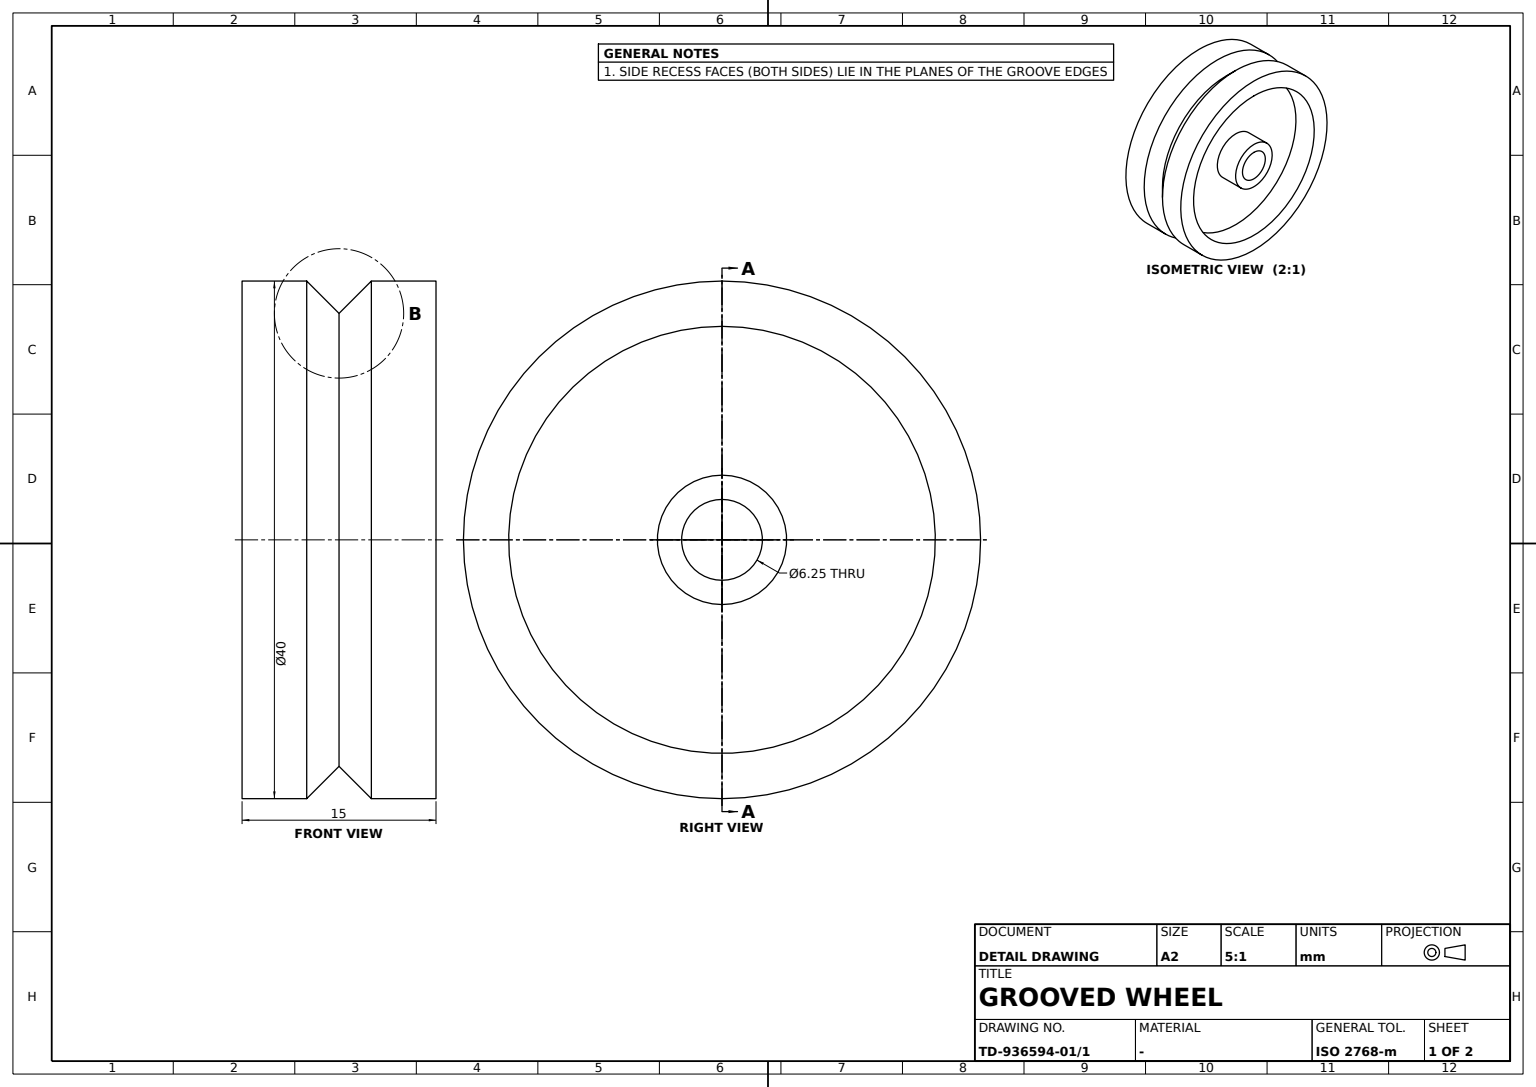
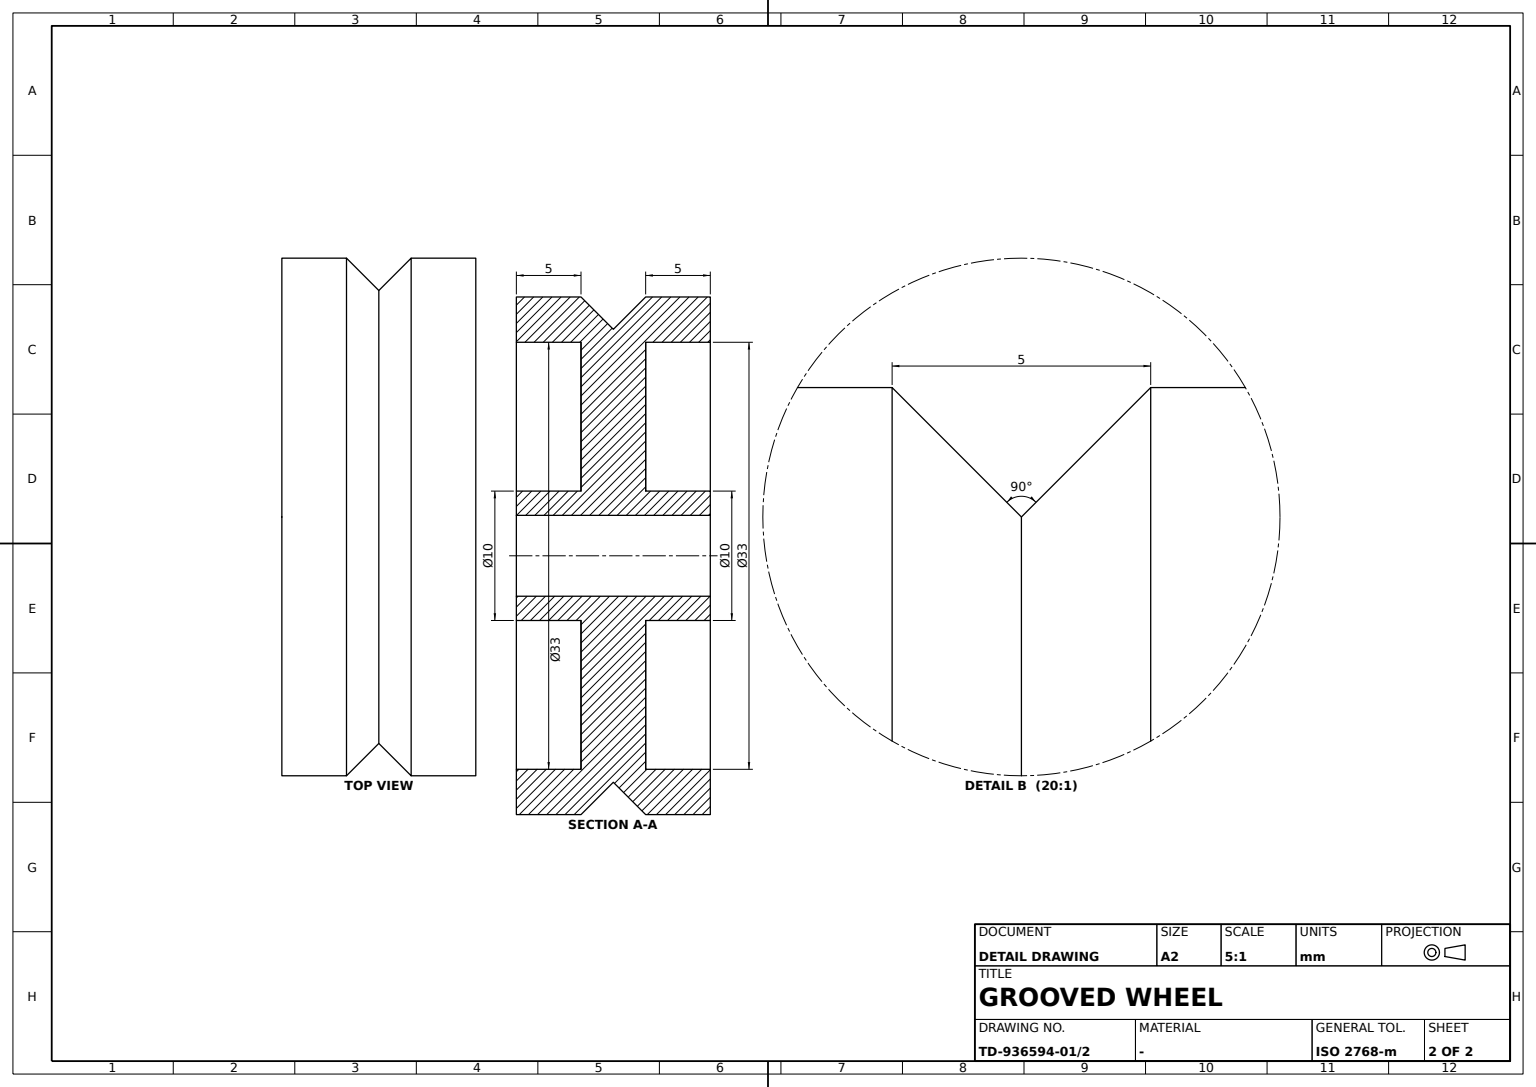
ISO-10303-21;
HEADER;
FILE_DESCRIPTION((''),'2;1');
FILE_NAME('','',(''),(''),'','','');
FILE_SCHEMA(('AUTOMOTIVE_DESIGN'));
ENDSEC;
DATA;
#1=APPLICATION_CONTEXT('');
#2=PRODUCT_CONTEXT('',#1,'mechanical');
#3=PRODUCT('','','',(#2));
#4=PRODUCT_DEFINITION_FORMATION('','',#3);
#5=PRODUCT_DEFINITION_CONTEXT('',#1,'design');
#6=PRODUCT_DEFINITION('','',#4,#5);
#7=PRODUCT_DEFINITION_SHAPE('','',#6);
#8=(LENGTH_UNIT()NAMED_UNIT(*)SI_UNIT(.MILLI.,.METRE.));
#9=(NAMED_UNIT(*)PLANE_ANGLE_UNIT()SI_UNIT($,.RADIAN.));
#10=(NAMED_UNIT(*)SI_UNIT($,.STERADIAN.)SOLID_ANGLE_UNIT());
#11=UNCERTAINTY_MEASURE_WITH_UNIT(LENGTH_MEASURE(0.005),#8,'distance_accuracy_value','');
#12=(GEOMETRIC_REPRESENTATION_CONTEXT(3)GLOBAL_UNCERTAINTY_ASSIGNED_CONTEXT((#11))GLOBAL_UNIT_ASSIGNED_CONTEXT((#8,#9,#10))REPRESENTATION_CONTEXT('',''));
#13=CARTESIAN_POINT('',(0.,2.5,20.));
#14=VERTEX_POINT('',#13);
#15=CARTESIAN_POINT('',(0.,2.5,0.));
#16=DIRECTION('',(0.,1.,0.));
#17=DIRECTION('',(0.,0.,1.));
#18=AXIS2_PLACEMENT_3D('',#15,#16,#17);
#19=CIRCLE('',#18,20.);
#20=EDGE_CURVE('',#14,#14,#19,.T.);
#21=ORIENTED_EDGE('',*,*,#20,.T.);
#22=EDGE_LOOP('',(#21));
#23=FACE_BOUND('',#22,.T.);
#24=CARTESIAN_POINT('',(0.,7.5,20.));
#25=VERTEX_POINT('',#24);
#26=CARTESIAN_POINT('',(0.,7.5,0.));
#27=AXIS2_PLACEMENT_3D('',#26,#16,#17);
#28=CIRCLE('',#27,20.);
#29=EDGE_CURVE('',#25,#25,#28,.T.);
#30=ORIENTED_EDGE('',*,*,#29,.F.);
#31=EDGE_LOOP('',(#30));
#32=FACE_BOUND('',#31,.T.);
#33=CARTESIAN_POINT('',(0.,0.,0.));
#34=DIRECTION('',(1.,0.,0.));
#35=AXIS2_PLACEMENT_3D('',#33,#16,#34);
#36=CYLINDRICAL_SURFACE('',#35,20.);
#37=ADVANCED_FACE('',(#23,#32),#36,.T.);
#38=CARTESIAN_POINT('',(0.,-7.5,3.125));
#39=VERTEX_POINT('',#38);
#40=CARTESIAN_POINT('',(0.,-7.5,0.));
#41=AXIS2_PLACEMENT_3D('',#40,#16,#17);
#42=CIRCLE('',#41,3.125);
#43=EDGE_CURVE('',#39,#39,#42,.T.);
#44=ORIENTED_EDGE('',*,*,#43,.F.);
#45=EDGE_LOOP('',(#44));
#46=FACE_BOUND('',#45,.T.);
#47=CARTESIAN_POINT('',(0.,7.5,3.125));
#48=VERTEX_POINT('',#47);
#49=CIRCLE('',#27,3.125);
#50=EDGE_CURVE('',#48,#48,#49,.T.);
#51=ORIENTED_EDGE('',*,*,#50,.T.);
#52=EDGE_LOOP('',(#51));
#53=FACE_BOUND('',#52,.T.);
#54=CARTESIAN_POINT('',(0.,-0.66,0.));
#55=DIRECTION('',(-1.,0.,0.));
#56=AXIS2_PLACEMENT_3D('',#54,#16,#55);
#57=CYLINDRICAL_SURFACE('',#56,3.125);
#58=ADVANCED_FACE('',(#46,#53),#57,.F.);
#59=CARTESIAN_POINT('',(0.,-7.5,20.));
#60=VERTEX_POINT('',#59);
#61=CIRCLE('',#41,20.);
#62=EDGE_CURVE('',#60,#60,#61,.T.);
#63=ORIENTED_EDGE('',*,*,#62,.T.);
#64=EDGE_LOOP('',(#63));
#65=FACE_BOUND('',#64,.T.);
#66=CARTESIAN_POINT('',(0.,-2.5,-20.));
#67=VERTEX_POINT('',#66);
#68=CARTESIAN_POINT('',(0.,-2.5,0.));
#69=DIRECTION('',(0.,-1.,0.));
#70=DIRECTION('',(0.,0.,-1.));
#71=AXIS2_PLACEMENT_3D('',#68,#69,#70);
#72=CIRCLE('',#71,20.);
#73=EDGE_CURVE('',#67,#67,#72,.F.);
#74=ORIENTED_EDGE('',*,*,#73,.F.);
#75=EDGE_LOOP('',(#74));
#76=FACE_BOUND('',#75,.T.);
#77=ADVANCED_FACE('',(#65,#76),#36,.T.);
#78=ORIENTED_EDGE('',*,*,#50,.F.);
#79=EDGE_LOOP('',(#78));
#80=FACE_BOUND('',#79,.T.);
#81=CARTESIAN_POINT('',(0.,7.5,5.));
#82=VERTEX_POINT('',#81);
#83=CIRCLE('',#27,5.);
#84=EDGE_CURVE('',#82,#82,#83,.T.);
#85=ORIENTED_EDGE('',*,*,#84,.T.);
#86=EDGE_LOOP('',(#85));
#87=FACE_BOUND('',#86,.T.);
#88=AXIS2_PLACEMENT_3D('',#26,#16,#34);
#89=PLANE('',#88);
#90=ADVANCED_FACE('',(#80,#87),#89,.T.);
#91=ORIENTED_EDGE('',*,*,#73,.T.);
#92=EDGE_LOOP('',(#91));
#93=FACE_BOUND('',#92,.T.);
#94=CARTESIAN_POINT('',(0.,0.,17.5));
#95=VERTEX_POINT('',#94);
#96=AXIS2_PLACEMENT_3D('',#33,#16,#17);
#97=CIRCLE('',#96,17.5);
#98=EDGE_CURVE('',#95,#95,#97,.T.);
#99=ORIENTED_EDGE('',*,*,#98,.F.);
#100=EDGE_LOOP('',(#99));
#101=FACE_BOUND('',#100,.T.);
#102=AXIS2_PLACEMENT_3D('',#33,#69,#34);
#103=CONICAL_SURFACE('',#102,17.5,0.785398163);
#104=ADVANCED_FACE('',(#93,#101),#103,.T.);
#105=ORIENTED_EDGE('',*,*,#20,.F.);
#106=EDGE_LOOP('',(#105));
#107=FACE_BOUND('',#106,.T.);
#108=ORIENTED_EDGE('',*,*,#98,.T.);
#109=EDGE_LOOP('',(#108));
#110=FACE_BOUND('',#109,.T.);
#111=CONICAL_SURFACE('',#35,17.5,0.785398163);
#112=ADVANCED_FACE('',(#107,#110),#111,.T.);
#113=CARTESIAN_POINT('',(0.,-2.5,16.5));
#114=VERTEX_POINT('',#113);
#115=AXIS2_PLACEMENT_3D('',#68,#16,#17);
#116=CIRCLE('',#115,16.5);
#117=EDGE_CURVE('',#114,#114,#116,.T.);
#118=ORIENTED_EDGE('',*,*,#117,.F.);
#119=EDGE_LOOP('',(#118));
#120=FACE_BOUND('',#119,.T.);
#121=CARTESIAN_POINT('',(0.,-2.5,5.));
#122=VERTEX_POINT('',#121);
#123=CIRCLE('',#115,5.);
#124=EDGE_CURVE('',#122,#122,#123,.T.);
#125=ORIENTED_EDGE('',*,*,#124,.T.);
#126=EDGE_LOOP('',(#125));
#127=FACE_BOUND('',#126,.T.);
#128=AXIS2_PLACEMENT_3D('',#121,#16,#34);
#129=PLANE('',#128);
#130=ADVANCED_FACE('',(#120,#127),#129,.F.);
#131=ORIENTED_EDGE('',*,*,#62,.F.);
#132=EDGE_LOOP('',(#131));
#133=FACE_BOUND('',#132,.T.);
#134=CARTESIAN_POINT('',(0.,-7.5,16.5));
#135=VERTEX_POINT('',#134);
#136=CIRCLE('',#41,16.5);
#137=EDGE_CURVE('',#135,#135,#136,.T.);
#138=ORIENTED_EDGE('',*,*,#137,.T.);
#139=EDGE_LOOP('',(#138));
#140=FACE_BOUND('',#139,.T.);
#141=AXIS2_PLACEMENT_3D('',#134,#16,#34);
#142=PLANE('',#141);
#143=ADVANCED_FACE('',(#133,#140),#142,.F.);
#144=CARTESIAN_POINT('',(0.,-7.5,5.));
#145=VERTEX_POINT('',#144);
#146=CIRCLE('',#41,5.);
#147=EDGE_CURVE('',#145,#145,#146,.T.);
#148=ORIENTED_EDGE('',*,*,#147,.T.);
#149=EDGE_LOOP('',(#148));
#150=FACE_BOUND('',#149,.T.);
#151=ORIENTED_EDGE('',*,*,#124,.F.);
#152=EDGE_LOOP('',(#151));
#153=FACE_BOUND('',#152,.T.);
#154=CYLINDRICAL_SURFACE('',#35,5.);
#155=ADVANCED_FACE('',(#150,#153),#154,.T.);
#156=CARTESIAN_POINT('',(0.,7.5,16.5));
#157=VERTEX_POINT('',#156);
#158=CIRCLE('',#27,16.5);
#159=EDGE_CURVE('',#157,#157,#158,.T.);
#160=ORIENTED_EDGE('',*,*,#159,.F.);
#161=EDGE_LOOP('',(#160));
#162=FACE_BOUND('',#161,.T.);
#163=ORIENTED_EDGE('',*,*,#29,.T.);
#164=EDGE_LOOP('',(#163));
#165=FACE_BOUND('',#164,.T.);
#166=ADVANCED_FACE('',(#162,#165),#89,.T.);
#167=ORIENTED_EDGE('',*,*,#84,.F.);
#168=EDGE_LOOP('',(#167));
#169=FACE_BOUND('',#168,.T.);
#170=CARTESIAN_POINT('',(0.,2.5,5.));
#171=VERTEX_POINT('',#170);
#172=CIRCLE('',#18,5.);
#173=EDGE_CURVE('',#171,#171,#172,.T.);
#174=ORIENTED_EDGE('',*,*,#173,.T.);
#175=EDGE_LOOP('',(#174));
#176=FACE_BOUND('',#175,.T.);
#177=ADVANCED_FACE('',(#169,#176),#154,.T.);
#178=ORIENTED_EDGE('',*,*,#117,.T.);
#179=EDGE_LOOP('',(#178));
#180=FACE_BOUND('',#179,.T.);
#181=ORIENTED_EDGE('',*,*,#137,.F.);
#182=EDGE_LOOP('',(#181));
#183=FACE_BOUND('',#182,.T.);
#184=CYLINDRICAL_SURFACE('',#35,16.5);
#185=ADVANCED_FACE('',(#180,#183),#184,.F.);
#186=ORIENTED_EDGE('',*,*,#159,.T.);
#187=EDGE_LOOP('',(#186));
#188=FACE_BOUND('',#187,.T.);
#189=CARTESIAN_POINT('',(0.,2.5,16.5));
#190=VERTEX_POINT('',#189);
#191=CIRCLE('',#18,16.5);
#192=EDGE_CURVE('',#190,#190,#191,.T.);
#193=ORIENTED_EDGE('',*,*,#192,.F.);
#194=EDGE_LOOP('',(#193));
#195=FACE_BOUND('',#194,.T.);
#196=ADVANCED_FACE('',(#188,#195),#184,.F.);
#197=ORIENTED_EDGE('',*,*,#173,.F.);
#198=EDGE_LOOP('',(#197));
#199=FACE_BOUND('',#198,.T.);
#200=ORIENTED_EDGE('',*,*,#192,.T.);
#201=EDGE_LOOP('',(#200));
#202=FACE_BOUND('',#201,.T.);
#203=AXIS2_PLACEMENT_3D('',#170,#16,#34);
#204=PLANE('',#203);
#205=ADVANCED_FACE('',(#199,#202),#204,.T.);
#206=ORIENTED_EDGE('',*,*,#147,.F.);
#207=EDGE_LOOP('',(#206));
#208=FACE_BOUND('',#207,.T.);
#209=ORIENTED_EDGE('',*,*,#43,.T.);
#210=EDGE_LOOP('',(#209));
#211=FACE_BOUND('',#210,.T.);
#212=ADVANCED_FACE('',(#208,#211),#142,.F.);
#213=CLOSED_SHELL('',(#37,#58,#77,#90,#104,#112,#130,#143,#155,#166,#177,#185,#196,#205,#212));
#214=MANIFOLD_SOLID_BREP('',#213);
#215=ADVANCED_BREP_SHAPE_REPRESENTATION('',(#214),#12);
#216=SHAPE_DEFINITION_REPRESENTATION(#7,#215);
ENDSEC;
END-ISO-10303-21;
